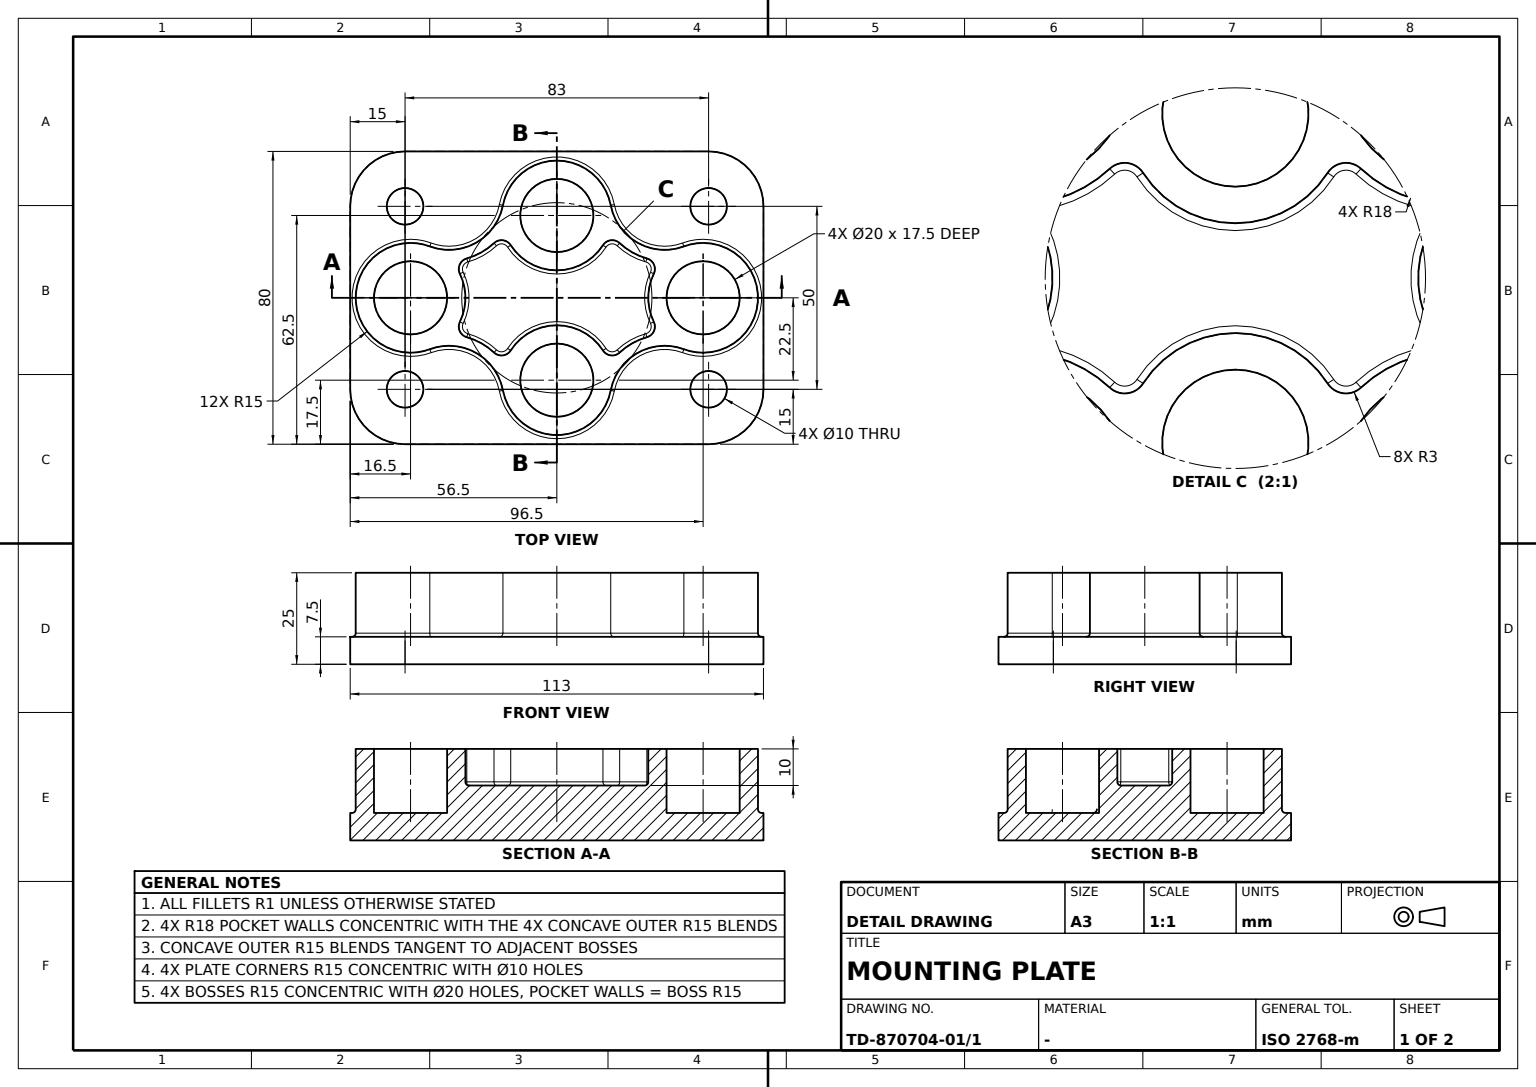
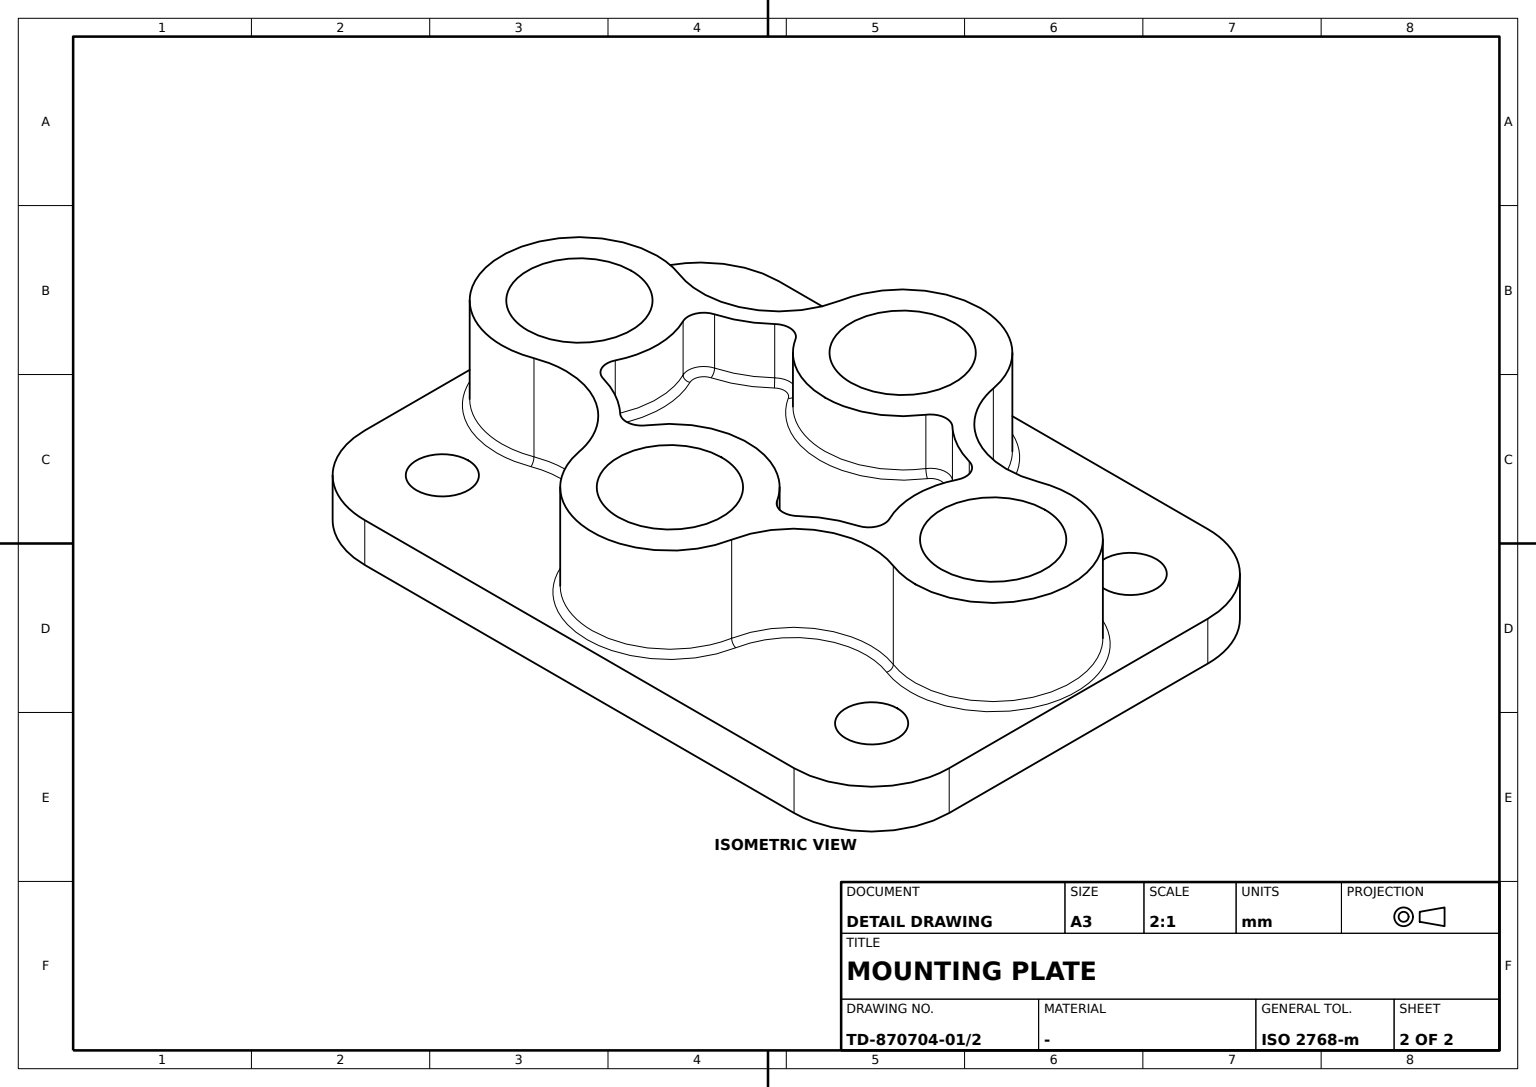
solid
v1 (-12.5,0,7.5)
v2 (-32.5,0,7.5)
e1 v1 v2 CIRCLE(AX(P(-22.5,0,7.5),D(0,0,-1),D(1,0,0)),10)
e2 v2 v1 CIRCLE(AX(P(-22.5,0,7.5),D(0,0,-1),D(1,0,0)),10)
face PLANE(AX(P(-22.5,0,7.5),D(0,0,1),D(1,0,0))) [-e1 -e2]
v3 (-14.213683,-16.498306,15)
v4 (-9.796458,-24.351149,15)
e3 v3 v4 CIRCLE(AX(P(-28.092789,-29.474069,15),D(0,0,-1),D(1,0,0)),19)
v5 (-14.944162,-17.181241,16)
e4 v5 v3 CIRCLE(AX(P(-14.213683,-16.498306,16),D(0.682934889,-0.730479252,0),D(0.730479252,0.682934889,0)),1)
v6 (-10.759423,-24.620776,16)
e5 v6 v5 CIRCLE(AX(P(-28.092789,-29.474069,16),D(0,0,1),D(1,0,0)),18)
e6 v6 v4 CIRCLE(AX(P(-9.796458,-24.351149,16),D(0.269627355,-0.962964739,0),D(0.962964739,0.269627355,0)),1)
face TORUS(AX(P(-28.092789,-29.474069,16),D(0,0,1),D(1,0,0)),19,1) rev [-e3 -e4 -e5 e6]
v7 (-6.996026,-25.610573,15)
v8 (6.996026,-25.610573,15)
e7 v7 v8 CIRCLE(AX(P(0,-40,15),D(0,0,-1),D(1,0,0)),16)
v9 (-6.558774,-26.509912,16)
e8 v9 v7 CIRCLE(AX(P(-6.996026,-25.610573,16),D(0.899339218,0.437251611,0),D(-0.437251611,0.899339218,0)),1)
v10 (6.558774,-26.509912,16)
e9 v10 v9 CIRCLE(AX(P(0,-40,16),D(0,0,1),D(1,0,0)),15)
e10 v10 v8 CIRCLE(AX(P(6.996026,-25.610573,16),D(0.899339218,-0.437251611,0),D(0.437251611,0.899339218,0)),1)
face TORUS(AX(P(0,-40,16),D(0,0,1),D(1,0,0)),16,1) rev [-e7 -e8 -e9 e10]
v11 (-25,56.5,0)
v12 (-25,56.5,7.5)
e11 v11 v12 LINE
v13 (25,56.5,7.5)
e12 v13 v12 LINE
v14 (25,56.5,0)
e13 v13 v14 LINE
e14 v14 v11 LINE
face PLANE(AX(P(40,56.5,7.5),D(0,-1,0),D(1,0,0))) rev [e11 -e12 e13 e14]
v15 (-10,40,25)
v16 (-10,40,7.5)
e15 v15 v16 LINE
v17 (10,40,25)
e16 v15 v17 CIRCLE(AX(P(0,40,25),D(0,0,1),D(1,0,0)),10)
v18 (10,40,7.5)
e17 v18 v17 LINE
e18 v18 v16 CIRCLE(AX(P(0,40,7.5),D(0,0,-1),D(1,0,0)),10)
face CYL(AX(P(0,40,7.5),D(0,0,1),D(1,0,0)),10) rev [-e15 e16 -e17 e18]
v19 (-40,-41.5,0)
v20 (-40,-41.5,7.5)
e19 v19 v20 LINE
v21 (-25,-56.5,0)
e20 v21 v19 CIRCLE(AX(P(-25,-41.5,0),D(0,0,-1),D(1,0,0)),15)
v22 (-25,-56.5,7.5)
e21 v22 v21 LINE
e22 v20 v22 CIRCLE(AX(P(-25,-41.5,7.5),D(0,0,1),D(1,0,0)),15)
face CYL(AX(P(-25,-41.5,7.5),D(0,0,-1),D(-1,0,0)),15) [-e19 -e20 -e21 -e22]
v23 (13.092789,-29.474069,8.5)
v24 (25.296394,-14.737034,8.5)
e23 v23 v24 CIRCLE(AX(P(28.092789,-29.474069,8.5),D(0,0,-1),D(1,0,0)),15)
v25 (25.296394,-14.737034,25)
e24 v25 v24 LINE
v26 (13.092789,-29.474069,25)
e25 v26 v25 CIRCLE(AX(P(28.092789,-29.474069,25),D(0,0,-1),D(-1,0,0)),15)
e26 v26 v23 LINE
face CYL(AX(P(28.092789,-29.474069,25),D(0,0,-1),D(-1,0,0)),15) rev [e23 -e24 -e25 e26]
v27 (-14.046394,34.737034,8.5)
v28 (-13.092789,29.474069,8.5)
e27 v27 v28 CIRCLE(AX(P(-28.092789,29.474069,8.5),D(0,0,-1),D(1,0,0)),15)
v29 (-25.296394,14.737034,8.5)
e28 v28 v29 CIRCLE(AX(P(-28.092789,29.474069,8.5),D(0,0,-1),D(1,0,0)),15)
v30 (-25.296394,14.737034,25)
e29 v30 v29 LINE
v31 (-14.046394,34.737034,25)
e30 v31 v30 CIRCLE(AX(P(-28.092789,29.474069,25),D(0,0,-1),D(-1,0,0)),15)
e31 v31 v27 LINE
face CYL(AX(P(-28.092789,29.474069,25),D(0,0,-1),D(-1,0,0)),15) rev [e27 e28 -e29 -e30 e31]
v32 (-20,-41.5,0)
v33 (-30,-41.5,0)
e32 v32 v33 CIRCLE(AX(P(-25,-41.5,0),D(0,0,1),D(-1,0,0)),5)
v34 (-20,-41.5,7.5)
e33 v32 v34 LINE
v35 (-30,-41.5,7.5)
e34 v34 v35 CIRCLE(AX(P(-25,-41.5,7.5),D(0,0,1),D(-1,0,0)),5)
e35 v35 v33 LINE
face CYL(AX(P(-25,-41.5,0),D(0,0,1),D(1,0,0)),5) rev [-e32 e33 e34 e35]
v36 (25.482821,-15.719503,7.5)
e36 v36 v24 CIRCLE(AX(P(25.482821,-15.719503,8.5),D(0.982468951,0.186426284,0),D(-0.186426284,0.982468951,0)),1)
v37 (38.5,0,7.5)
e37 v37 v36 CIRCLE(AX(P(22.5,0,7.5),D(0,0,-1),D(1,0,0)),16)
v38 (37.5,0,8.5)
e38 v38 v37 CIRCLE(AX(P(38.5,0,8.5),D(0,-1,0),D(0,0,-1)),1)
e39 v24 v38 CIRCLE(AX(P(22.5,0,8.5),D(0,0,1),D(1,0,0)),15)
face TORUS(AX(P(22.5,0,8.5),D(0,0,1),D(1,0,0)),16,1) rev [-e36 -e37 -e38 -e39]
v39 (-15,-40,8.5)
v40 (15,-40,8.5)
e40 v39 v40 CIRCLE(AX(P(0,-40,8.5),D(0,0,1),D(1,0,0)),15)
v41 (-16,-40,7.5)
e41 v39 v41 CIRCLE(AX(P(-16,-40,8.5),D(0,1,0),D(-1,0,0)),1)
v42 (16,-40,7.5)
e42 v42 v41 CIRCLE(AX(P(0,-40,7.5),D(0,0,-1),D(1,0,0)),16)
e43 v40 v42 CIRCLE(AX(P(16,-40,8.5),D(0,-1,0),D(0,0,-1)),1)
face TORUS(AX(P(0,-40,8.5),D(0,0,1),D(1,0,0)),16,1) rev [-e40 e41 -e42 -e43]
v43 (30,41.5,7.5)
v44 (20,41.5,7.5)
e44 v43 v44 CIRCLE(AX(P(25,41.5,7.5),D(0,0,1),D(-1,0,0)),5)
e45 v44 v43 CIRCLE(AX(P(25,41.5,7.5),D(0,0,1),D(-1,0,0)),5)
v45 (30,-41.5,7.5)
v46 (20,-41.5,7.5)
e46 v45 v46 CIRCLE(AX(P(25,-41.5,7.5),D(0,0,1),D(-1,0,0)),5)
e47 v46 v45 CIRCLE(AX(P(25,-41.5,7.5),D(0,0,1),D(-1,0,0)),5)
v47 (25,-56.5,7.5)
v48 (40,-41.5,7.5)
e48 v47 v48 CIRCLE(AX(P(25,-41.5,7.5),D(0,0,1),D(1,0,0)),15)
v49 (40,41.5,7.5)
e49 v48 v49 LINE
e50 v49 v13 CIRCLE(AX(P(25,41.5,7.5),D(0,0,1),D(1,0,0)),15)
v50 (-40,41.5,7.5)
e51 v12 v50 CIRCLE(AX(P(-25,41.5,7.5),D(0,0,1),D(1,0,0)),15)
e52 v50 v20 LINE
e53 v22 v47 LINE
v51 (-20,41.5,7.5)
v52 (-30,41.5,7.5)
e54 v51 v52 CIRCLE(AX(P(-25,41.5,7.5),D(0,0,1),D(-1,0,0)),5)
e55 v52 v51 CIRCLE(AX(P(-25,41.5,7.5),D(0,0,1),D(-1,0,0)),5)
e56 v35 v34 CIRCLE(AX(P(-25,-41.5,7.5),D(0,0,1),D(-1,0,0)),5)
v53 (16,40,7.5)
v54 (14.982821,34.38617,7.5)
e57 v53 v54 CIRCLE(AX(P(0,40,7.5),D(0,0,-1),D(1,0,0)),16)
v55 (25.482821,15.719503,7.5)
e58 v54 v55 CIRCLE(AX(P(28.092789,29.474069,7.5),D(0,0,1),D(1,0,0)),14)
e59 v55 v37 CIRCLE(AX(P(22.5,0,7.5),D(0,0,-1),D(1,0,0)),16)
v56 (14.982821,-34.38617,7.5)
e60 v36 v56 CIRCLE(AX(P(28.092789,-29.474069,7.5),D(0,0,1),D(1,0,0)),14)
e61 v56 v42 CIRCLE(AX(P(0,-40,7.5),D(0,0,-1),D(1,0,0)),16)
v57 (-14.982821,-34.38617,7.5)
e62 v41 v57 CIRCLE(AX(P(0,-40,7.5),D(0,0,-1),D(1,0,0)),16)
v58 (-14.092789,-29.474069,7.5)
e63 v57 v58 CIRCLE(AX(P(-28.092789,-29.474069,7.5),D(0,0,1),D(1,0,0)),14)
v59 (-25.482821,-15.719503,7.5)
e64 v58 v59 CIRCLE(AX(P(-28.092789,-29.474069,7.5),D(0,0,1),D(1,0,0)),14)
v60 (-25.482821,15.719503,7.5)
e65 v59 v60 CIRCLE(AX(P(-22.5,0,7.5),D(0,0,-1),D(1,0,0)),16)
v61 (-14.092789,29.474069,7.5)
e66 v60 v61 CIRCLE(AX(P(-28.092789,29.474069,7.5),D(0,0,1),D(1,0,0)),14)
v62 (-14.982821,34.38617,7.5)
e67 v61 v62 CIRCLE(AX(P(-28.092789,29.474069,7.5),D(0,0,1),D(1,0,0)),14)
v63 (-16,40,7.5)
e68 v62 v63 CIRCLE(AX(P(0,40,7.5),D(0,0,-1),D(1,0,0)),16)
e69 v63 v53 CIRCLE(AX(P(0,40,7.5),D(0,0,-1),D(1,0,0)),16)
face PLANE(AX(P(0,0,7.5),D(0,0,1),D(1,0,0))) [-e44 -e45] [-e46 -e47] [e48 e49 e50 e12 e51 e52 e22 e53] [-e54 -e55] [-e34 -e56] [e57 e58 e59 e37 e60 e61 e42 e62 e63 e64 e65 e66 e67 e68 e69]
v64 (-20,41.5,0)
e70 v64 v51 LINE
v65 (-30,41.5,0)
e71 v65 v64 CIRCLE(AX(P(-25,41.5,0),D(0,0,1),D(-1,0,0)),5)
e72 v52 v65 LINE
face CYL(AX(P(-25,41.5,0),D(0,0,1),D(1,0,0)),5) rev [-e70 -e71 -e72 e55]
v66 (14.37727,-12.610363,16)
v67 (15.752724,-15.132436,16)
e73 v66 v67 CIRCLE(AX(P(12.752724,-15.132436,16),D(0,0,-1),D(1,0,0)),3)
v68 (15.752724,-15.132436,25)
e74 v67 v68 LINE
v69 (14.37727,-12.610363,25)
e75 v68 v69 CIRCLE(AX(P(12.752724,-15.132436,25),D(0,0,1),D(1,0,0)),3)
e76 v69 v66 LINE
face CYL(AX(P(12.752724,-15.132436,15),D(0,0,1),D(1,0,0)),3) rev [e73 e74 e75 e76]
v70 (10.759423,-24.620776,25)
v71 (14.944162,-17.181241,25)
e77 v70 v71 CIRCLE(AX(P(28.092789,-29.474069,25),D(0,0,-1),D(1,0,0)),18)
v72 (14.944162,-17.181241,16)
e78 v71 v72 LINE
v73 (10.759423,-24.620776,16)
e79 v72 v73 CIRCLE(AX(P(28.092789,-29.474069,16),D(0,0,1),D(1,0,0)),18)
e80 v70 v73 LINE
face CYL(AX(P(28.092789,-29.474069,15),D(0,0,1),D(1,0,0)),18) [e77 e78 e79 -e80]
v74 (15,40,8.5)
v75 (-15,40,8.5)
e81 v74 v75 CIRCLE(AX(P(0,40,8.5),D(0,0,1),D(1,0,0)),15)
e82 v74 v53 CIRCLE(AX(P(16,40,8.5),D(0,-1,0),D(0,0,-1)),1)
e83 v75 v63 CIRCLE(AX(P(-16,40,8.5),D(0,1,0),D(-1,0,0)),1)
face TORUS(AX(P(0,40,8.5),D(0,0,1),D(1,0,0)),16,1) rev [-e81 e82 -e69 -e83]
v76 (-37.5,0,8.5)
e84 v29 v76 CIRCLE(AX(P(-22.5,0,8.5),D(0,0,1),D(1,0,0)),15)
v77 (-37.5,0,25)
e85 v77 v76 LINE
e86 v30 v77 CIRCLE(AX(P(-22.5,0,25),D(0,0,1),D(-1,0,0)),15)
face CYL(AX(P(-22.5,0,25),D(0,0,-1),D(-1,0,0)),15) [e84 -e85 -e86 e29]
v78 (-15,-40,25)
e87 v78 v39 LINE
v79 (15,-40,25)
e88 v79 v40 LINE
e89 v78 v79 CIRCLE(AX(P(0,-40,25),D(0,0,1),D(-1,0,0)),15)
face CYL(AX(P(0,-40,25),D(0,0,-1),D(-1,0,0)),15) [e87 e40 -e88 -e89]
v80 (-10,-40,25)
v81 (-10,-40,7.5)
e90 v80 v81 LINE
v82 (10,-40,7.5)
e91 v81 v82 CIRCLE(AX(P(0,-40,7.5),D(0,0,-1),D(1,0,0)),10)
v83 (10,-40,25)
e92 v82 v83 LINE
e93 v83 v80 CIRCLE(AX(P(0,-40,25),D(0,0,1),D(1,0,0)),10)
face CYL(AX(P(0,-40,7.5),D(0,0,1),D(1,0,0)),10) rev [e90 e91 e92 e93]
e94 v33 v32 CIRCLE(AX(P(-25,-41.5,0),D(0,0,1),D(-1,0,0)),5)
face CYL(AX(P(-25,-41.5,0),D(0,0,1),D(1,0,0)),5) rev [-e94 -e35 e56 -e33]
v84 (10.759423,24.620776,16)
v85 (14.944162,17.181241,16)
e95 v84 v85 CIRCLE(AX(P(28.092789,29.474069,16),D(0,0,1),D(1,0,0)),18)
v86 (9.796458,24.351149,15)
e96 v86 v84 CIRCLE(AX(P(9.796458,24.351149,16),D(0.269627355,-0.962964739,0),D(0.962964739,0.269627355,0)),1)
v87 (14.213683,16.498306,15)
e97 v87 v86 CIRCLE(AX(P(28.092789,29.474069,15),D(0,0,-1),D(1,0,0)),19)
e98 v87 v85 CIRCLE(AX(P(14.213683,16.498306,16),D(0.682934889,-0.730479252,0),D(0.730479252,0.682934889,0)),1)
face TORUS(AX(P(28.092789,29.474069,16),D(0,0,1),D(1,0,0)),19,1) rev [-e95 -e96 -e97 e98]
e99 v62 v27 CIRCLE(AX(P(-14.982821,34.38617,8.5),D(0.350864382,-0.936426284,0),D(0.936426284,0.350864382,0)),1)
e100 v75 v27 CIRCLE(AX(P(0,40,8.5),D(0,0,1),D(1,0,0)),15)
face TORUS(AX(P(0,40,8.5),D(0,0,1),D(1,0,0)),16,1) rev [e83 -e68 e99 -e100]
e101 v61 v28 CIRCLE(AX(P(-14.092789,29.474069,8.5),D(0,-1,0),D(0,0,-1)),1)
e102 v29 v60 CIRCLE(AX(P(-25.482821,15.719503,8.5),D(0.982468951,0.186426284,0),D(-0.186426284,0.982468951,0)),1)
face TORUS(AX(P(-28.092789,29.474069,8.5),D(0,0,1),D(1,0,0)),14,1) rev [-e101 -e66 -e102 -e28]
v88 (40,-41.5,0)
e103 v48 v88 LINE
v89 (40,41.5,0)
e104 v88 v89 LINE
e105 v89 v49 LINE
face PLANE(AX(P(40,-56.5,7.5),D(-1,0,0),D(0,-1,0))) rev [e103 e104 e105 -e49]
e106 v80 v83 CIRCLE(AX(P(0,-40,25),D(0,0,1),D(1,0,0)),10)
e107 v82 v81 CIRCLE(AX(P(0,-40,7.5),D(0,0,-1),D(1,0,0)),10)
face CYL(AX(P(0,-40,7.5),D(0,0,1),D(1,0,0)),10) rev [-e90 e106 -e92 e107]
v90 (-6.558774,26.509912,16)
v91 (6.558774,26.509912,16)
e108 v90 v91 CIRCLE(AX(P(0,40,16),D(0,0,1),D(1,0,0)),15)
v92 (-6.996026,25.610573,15)
e109 v92 v90 CIRCLE(AX(P(-6.996026,25.610573,16),D(0.899339218,-0.437251611,0),D(0.437251611,0.899339218,0)),1)
v93 (6.996026,25.610573,15)
e110 v93 v92 CIRCLE(AX(P(0,40,15),D(0,0,-1),D(1,0,0)),16)
e111 v93 v91 CIRCLE(AX(P(6.996026,25.610573,16),D(0.899339218,0.437251611,0),D(-0.437251611,0.899339218,0)),1)
face TORUS(AX(P(0,40,16),D(0,0,1),D(1,0,0)),16,1) rev [-e108 -e109 -e110 e111]
v94 (20,41.5,0)
e112 v44 v94 LINE
v95 (30,41.5,0)
e113 v95 v43 LINE
e114 v94 v95 CIRCLE(AX(P(25,41.5,0),D(0,0,1),D(-1,0,0)),5)
face CYL(AX(P(25,41.5,0),D(0,0,1),D(1,0,0)),5) rev [-e112 e45 -e113 -e114]
v96 (-40,41.5,0)
e115 v50 v96 LINE
e116 v96 v19 LINE
face PLANE(AX(P(-40,56.5,7.5),D(1,0,0),D(0,1,0))) rev [-e52 e115 e116 e19]
v97 (14.046394,-34.737034,8.5)
e117 v97 v23 CIRCLE(AX(P(28.092789,-29.474069,8.5),D(0,0,-1),D(1,0,0)),15)
e118 v97 v56 CIRCLE(AX(P(14.982821,-34.38617,8.5),D(0.350864382,-0.936426284,0),D(0.936426284,0.350864382,0)),1)
face TORUS(AX(P(28.092789,-29.474069,8.5),D(0,0,1),D(1,0,0)),14,1) rev [-e60 e36 -e23 -e117 e118]
v98 (6.558774,26.509912,25)
e119 v98 v91 LINE
v99 (-6.558774,26.509912,25)
e120 v98 v99 CIRCLE(AX(P(0,40,25),D(0,0,-1),D(1,0,0)),15)
e121 v99 v90 LINE
face CYL(AX(P(0,40,15),D(0,0,1),D(1,0,0)),15) [-e119 e120 e121 e108]
v100 (-7.5,0,16)
v101 (-7.5,0,25)
e122 v100 v101 LINE
v102 (-14.37727,12.610363,16)
e123 v100 v102 CIRCLE(AX(P(-22.5,0,16),D(0,0,1),D(1,0,0)),15)
v103 (-14.37727,12.610363,25)
e124 v103 v102 LINE
e125 v103 v101 CIRCLE(AX(P(-22.5,0,25),D(0,0,-1),D(1,0,0)),15)
face CYL(AX(P(-22.5,0,15),D(0,0,1),D(1,0,0)),15) [-e122 e123 -e124 e125]
v104 (12.5,0,25)
v105 (32.5,0,25)
e126 v104 v105 CIRCLE(AX(P(22.5,0,25),D(0,0,1),D(1,0,0)),10)
e127 v105 v104 CIRCLE(AX(P(22.5,0,25),D(0,0,1),D(1,0,0)),10)
v106 (-14.046394,-34.737034,25)
e128 v106 v78 CIRCLE(AX(P(0,-40,25),D(0,0,1),D(-1,0,0)),15)
v107 (14.046394,-34.737034,25)
e129 v79 v107 CIRCLE(AX(P(0,-40,25),D(0,0,1),D(-1,0,0)),15)
e130 v107 v26 CIRCLE(AX(P(28.092789,-29.474069,25),D(0,0,-1),D(-1,0,0)),15)
v108 (25.296394,14.737034,25)
e131 v25 v108 CIRCLE(AX(P(22.5,0,25),D(0,0,1),D(-1,0,0)),15)
v109 (13.092789,29.474069,25)
e132 v108 v109 CIRCLE(AX(P(28.092789,29.474069,25),D(0,0,-1),D(-1,0,0)),15)
v110 (14.046394,34.737034,25)
e133 v109 v110 CIRCLE(AX(P(28.092789,29.474069,25),D(0,0,-1),D(-1,0,0)),15)
v111 (15,40,25)
e134 v110 v111 CIRCLE(AX(P(0,40,25),D(0,0,1),D(-1,0,0)),15)
v112 (-15,40,25)
e135 v111 v112 CIRCLE(AX(P(0,40,25),D(0,0,1),D(-1,0,0)),15)
e136 v112 v31 CIRCLE(AX(P(0,40,25),D(0,0,1),D(-1,0,0)),15)
v113 (-25.296394,-14.737034,25)
e137 v77 v113 CIRCLE(AX(P(-22.5,0,25),D(0,0,1),D(-1,0,0)),15)
e138 v113 v106 CIRCLE(AX(P(-28.092789,-29.474069,25),D(0,0,-1),D(-1,0,0)),15)
v114 (15.752724,15.132436,25)
v115 (14.944162,17.181241,25)
e139 v114 v115 CIRCLE(AX(P(12.752724,15.132436,25),D(0,0,1),D(1,0,0)),3)
v116 (14.37727,12.610363,25)
e140 v116 v114 CIRCLE(AX(P(12.752724,15.132436,25),D(0,0,1),D(1,0,0)),3)
e141 v69 v116 CIRCLE(AX(P(22.5,0,25),D(0,0,-1),D(1,0,0)),15)
e142 v71 v68 CIRCLE(AX(P(12.752724,-15.132436,25),D(0,0,1),D(1,0,0)),3)
v117 (6.558774,-26.509912,25)
e143 v117 v70 CIRCLE(AX(P(7.870529,-23.811894,25),D(0,0,1),D(1,0,0)),3)
v118 (-6.558774,-26.509912,25)
e144 v118 v117 CIRCLE(AX(P(0,-40,25),D(0,0,-1),D(1,0,0)),15)
v119 (-10.759423,-24.620776,25)
e145 v119 v118 CIRCLE(AX(P(-7.870529,-23.811894,25),D(0,0,1),D(1,0,0)),3)
v120 (-14.944162,-17.181241,25)
e146 v120 v119 CIRCLE(AX(P(-28.092789,-29.474069,25),D(0,0,-1),D(1,0,0)),18)
v121 (-14.37727,-12.610363,25)
e147 v121 v120 CIRCLE(AX(P(-12.752724,-15.132436,25),D(0,0,1),D(1,0,0)),3)
e148 v101 v121 CIRCLE(AX(P(-22.5,0,25),D(0,0,-1),D(1,0,0)),15)
v122 (-14.944162,17.181241,25)
e149 v122 v103 CIRCLE(AX(P(-12.752724,15.132436,25),D(0,0,1),D(1,0,0)),3)
v123 (-10.759423,24.620776,25)
e150 v123 v122 CIRCLE(AX(P(-28.092789,29.474069,25),D(0,0,-1),D(1,0,0)),18)
e151 v99 v123 CIRCLE(AX(P(-7.870529,23.811894,25),D(0,0,1),D(1,0,0)),3)
v124 (10.759423,24.620776,25)
e152 v124 v98 CIRCLE(AX(P(7.870529,23.811894,25),D(0,0,1),D(1,0,0)),3)
e153 v115 v124 CIRCLE(AX(P(28.092789,29.474069,25),D(0,0,-1),D(1,0,0)),18)
v125 (-32.5,0,25)
v126 (-12.5,0,25)
e154 v125 v126 CIRCLE(AX(P(-22.5,0,25),D(0,0,1),D(1,0,0)),10)
e155 v126 v125 CIRCLE(AX(P(-22.5,0,25),D(0,0,1),D(1,0,0)),10)
e156 v17 v15 CIRCLE(AX(P(0,40,25),D(0,0,1),D(1,0,0)),10)
face PLANE(AX(P(-25.296394,-14.737034,25),D(0,0,1),D(1,0,0))) [-e126 -e127] [e128 e89 e129 e130 e25 e131 e132 e133 e134 e135 e136 e30 e86 e137 e138] [-e139 -e140 -e141 -e75 -e142 -e77 -e143 -e144 -e145 -e146 -e147 -e148 -e125 -e149 -e150 -e151 -e120 -e152 -e153] [-e154 -e155] [-e93 -e106] [-e156 -e16]
e157 v16 v18 CIRCLE(AX(P(0,40,7.5),D(0,0,-1),D(1,0,0)),10)
face PLANE(AX(P(0,40,7.5),D(0,0,1),D(1,0,0))) [-e18 -e157]
v127 (-14.213683,16.498306,15)
v128 (-14.944162,17.181241,16)
e158 v127 v128 CIRCLE(AX(P(-14.213683,16.498306,16),D(0.682934889,0.730479252,0),D(-0.730479252,0.682934889,0)),1)
e159 v102 v128 CIRCLE(AX(P(-12.752724,15.132436,16),D(0,0,-1),D(1,0,0)),3)
v129 (-13.835755,13.451054,15)
e160 v102 v129 CIRCLE(AX(P(-13.835755,13.451054,16),D(0.840690882,-0.54151532,0),D(0.54151532,0.840690882,0)),1)
e161 v127 v129 CIRCLE(AX(P(-12.752724,15.132436,15),D(0,0,1),D(1,0,0)),2)
face TORUS(AX(P(-12.752724,15.132436,16),D(0,0,1),D(1,0,0)),2,1) rev [e158 -e159 e160 -e161]
e162 v64 v65 CIRCLE(AX(P(-25,41.5,0),D(0,0,1),D(-1,0,0)),5)
face CYL(AX(P(-25,41.5,0),D(0,0,1),D(1,0,0)),5) rev [-e162 e70 e54 e72]
v130 (13.835755,13.451054,15)
v131 (14.37727,12.610363,16)
e163 v130 v131 CIRCLE(AX(P(13.835755,13.451054,16),D(-0.840690882,-0.54151532,0),D(0.54151532,-0.840690882,0)),1)
v132 (15.752724,15.132436,16)
e164 v132 v131 CIRCLE(AX(P(12.752724,15.132436,16),D(0,0,-1),D(1,0,0)),3)
v133 (14.752724,15.132436,15)
e165 v133 v132 CIRCLE(AX(P(14.752724,15.132436,16),D(0,-1,0),D(0,0,-1)),1)
e166 v130 v133 CIRCLE(AX(P(12.752724,15.132436,15),D(0,0,1),D(1,0,0)),2)
face TORUS(AX(P(12.752724,15.132436,16),D(0,0,1),D(1,0,0)),2,1) rev [e163 -e164 -e165 -e166]
v134 (-10.759423,24.620776,16)
e167 v123 v134 LINE
e168 v134 v90 CIRCLE(AX(P(-7.870529,23.811894,16),D(0,0,-1),D(1,0,0)),3)
face CYL(AX(P(-7.870529,23.811894,15),D(0,0,1),D(1,0,0)),3) rev [e151 e167 e168 -e121]
e169 v117 v10 LINE
e170 v73 v10 CIRCLE(AX(P(7.870529,-23.811894,16),D(0,0,-1),D(1,0,0)),3)
face CYL(AX(P(7.870529,-23.811894,15),D(0,0,1),D(1,0,0)),3) rev [-e169 e143 e80 e170]
v135 (-14.046394,-34.737034,8.5)
e171 v106 v135 LINE
e172 v135 v39 CIRCLE(AX(P(0,-40,8.5),D(0,0,1),D(1,0,0)),15)
face CYL(AX(P(0,-40,25),D(0,0,-1),D(-1,0,0)),15) [-e87 -e128 e171 e172]
e173 v125 v2 LINE
e174 v1 v126 LINE
face CYL(AX(P(-22.5,0,7.5),D(0,0,1),D(1,0,0)),10) rev [e173 e2 e174 e155]
e175 v112 v75 LINE
e176 v111 v74 LINE
face CYL(AX(P(0,40,25),D(0,0,-1),D(-1,0,0)),15) [e81 -e175 -e135 e176]
v136 (-9.796458,24.351149,15)
e177 v136 v134 CIRCLE(AX(P(-9.796458,24.351149,16),D(0.269627355,0.962964739,0),D(-0.962964739,0.269627355,0)),1)
e178 v92 v136 CIRCLE(AX(P(-7.870529,23.811894,15),D(0,0,1),D(1,0,0)),2)
face TORUS(AX(P(-7.870529,23.811894,16),D(0,0,1),D(1,0,0)),2,1) rev [e109 -e168 -e177 -e178]
e179 v132 v114 LINE
e180 v116 v131 LINE
face CYL(AX(P(12.752724,15.132436,15),D(0,0,1),D(1,0,0)),3) rev [e140 -e179 e164 -e180]
v137 (-14.37727,-12.610363,16)
v138 (-13.835755,-13.451054,15)
e181 v137 v138 CIRCLE(AX(P(-13.835755,-13.451054,16),D(-0.840690882,-0.54151532,0),D(0.54151532,-0.840690882,0)),1)
e182 v5 v137 CIRCLE(AX(P(-12.752724,-15.132436,16),D(0,0,-1),D(1,0,0)),3)
e183 v138 v3 CIRCLE(AX(P(-12.752724,-15.132436,15),D(0,0,1),D(1,0,0)),2)
face TORUS(AX(P(-12.752724,-15.132436,16),D(0,0,1),D(1,0,0)),2,1) rev [-e181 -e182 e4 -e183]
e184 v86 v93 CIRCLE(AX(P(7.870529,23.811894,15),D(0,0,1),D(1,0,0)),2)
e185 v91 v84 CIRCLE(AX(P(7.870529,23.811894,16),D(0,0,-1),D(1,0,0)),3)
face TORUS(AX(P(7.870529,23.811894,16),D(0,0,1),D(1,0,0)),2,1) rev [-e111 -e184 e96 -e185]
v139 (-6.5,0,15)
e186 v100 v139 CIRCLE(AX(P(-6.5,0,16),D(0,-1,0),D(0,0,-1)),1)
e187 v129 v139 CIRCLE(AX(P(-22.5,0,15),D(0,0,-1),D(1,0,0)),16)
face TORUS(AX(P(-22.5,0,16),D(0,0,1),D(1,0,0)),16,1) rev [-e123 e186 -e187 -e160]
v140 (14.046394,34.737034,8.5)
e188 v54 v140 CIRCLE(AX(P(14.982821,34.38617,8.5),D(0.350864382,0.936426284,0),D(-0.936426284,0.350864382,0)),1)
v141 (13.092789,29.474069,8.5)
e189 v141 v140 CIRCLE(AX(P(28.092789,29.474069,8.5),D(0,0,-1),D(1,0,0)),15)
v142 (25.296394,14.737034,8.5)
e190 v142 v141 CIRCLE(AX(P(28.092789,29.474069,8.5),D(0,0,-1),D(1,0,0)),15)
e191 v55 v142 CIRCLE(AX(P(25.482821,15.719503,8.5),D(-0.982468951,0.186426284,0),D(-0.186426284,-0.982468951,0)),1)
face TORUS(AX(P(28.092789,29.474069,8.5),D(0,0,1),D(1,0,0)),14,1) rev [e188 -e189 -e190 -e191 -e58]
face CYL(AX(P(-22.5,0,7.5),D(0,0,1),D(1,0,0)),10) rev [e154 -e174 e1 -e173]
e192 v115 v85 LINE
e193 v85 v132 CIRCLE(AX(P(12.752724,15.132436,16),D(0,0,-1),D(1,0,0)),3)
face CYL(AX(P(12.752724,15.132436,15),D(0,0,1),D(1,0,0)),3) rev [e179 e139 e192 e193]
v143 (20,-41.5,0)
e194 v46 v143 LINE
v144 (30,-41.5,0)
e195 v144 v143 CIRCLE(AX(P(25,-41.5,0),D(0,0,1),D(-1,0,0)),5)
e196 v144 v45 LINE
face CYL(AX(P(25,-41.5,0),D(0,0,1),D(1,0,0)),5) rev [e46 e194 -e195 e196]
e197 v40 v97 CIRCLE(AX(P(0,-40,8.5),D(0,0,1),D(1,0,0)),15)
face TORUS(AX(P(0,-40,8.5),D(0,0,1),D(1,0,0)),16,1) rev [-e118 -e197 e43 -e61]
v145 (-25.296394,-14.737034,8.5)
v146 (-13.092789,-29.474069,8.5)
e198 v145 v146 CIRCLE(AX(P(-28.092789,-29.474069,8.5),D(0,0,-1),D(1,0,0)),15)
e199 v145 v59 CIRCLE(AX(P(-25.482821,-15.719503,8.5),D(-0.982468951,0.186426284,0),D(-0.186426284,-0.982468951,0)),1)
e200 v58 v146 CIRCLE(AX(P(-14.092789,-29.474069,8.5),D(0,-1,0),D(0,0,-1)),1)
face TORUS(AX(P(-28.092789,-29.474069,8.5),D(0,0,1),D(1,0,0)),14,1) rev [-e198 e199 -e64 e200]
e201 v107 v97 LINE
face CYL(AX(P(0,-40,25),D(0,0,-1),D(-1,0,0)),15) [-e129 e88 e197 -e201]
e202 v76 v145 CIRCLE(AX(P(-22.5,0,8.5),D(0,0,1),D(1,0,0)),15)
face TORUS(AX(P(-22.5,0,8.5),D(0,0,1),D(1,0,0)),16,1) rev [-e84 e102 -e65 -e199 -e202]
e203 v121 v137 LINE
e204 v137 v100 CIRCLE(AX(P(-22.5,0,16),D(0,0,1),D(1,0,0)),15)
face CYL(AX(P(-22.5,0,15),D(0,0,1),D(1,0,0)),15) [e148 e203 e204 e122]
e205 v38 v142 CIRCLE(AX(P(22.5,0,8.5),D(0,0,1),D(1,0,0)),15)
face TORUS(AX(P(22.5,0,8.5),D(0,0,1),D(1,0,0)),16,1) rev [e191 -e205 e38 -e59]
face CYL(AX(P(28.092789,-29.474069,25),D(0,0,-1),D(-1,0,0)),15) rev [-e26 -e130 e201 e117]
v147 (14.213683,-16.498306,15)
e206 v72 v147 CIRCLE(AX(P(14.213683,-16.498306,16),D(0.682934889,0.730479252,0),D(-0.730479252,0.682934889,0)),1)
v148 (9.796458,-24.351149,15)
e207 v148 v147 CIRCLE(AX(P(28.092789,-29.474069,15),D(0,0,-1),D(1,0,0)),19)
e208 v73 v148 CIRCLE(AX(P(9.796458,-24.351149,16),D(0.269627355,0.962964739,0),D(-0.962964739,0.269627355,0)),1)
face TORUS(AX(P(28.092789,-29.474069,16),D(0,0,1),D(1,0,0)),19,1) rev [e206 -e207 -e208 -e79]
e209 v113 v145 LINE
face CYL(AX(P(-22.5,0,25),D(0,0,-1),D(-1,0,0)),15) [-e137 e85 e202 -e209]
e210 v95 v94 CIRCLE(AX(P(25,41.5,0),D(0,0,1),D(-1,0,0)),5)
face CYL(AX(P(25,41.5,0),D(0,0,1),D(1,0,0)),5) rev [-e210 e113 e44 e112]
e211 v139 v138 CIRCLE(AX(P(-22.5,0,15),D(0,0,-1),D(1,0,0)),16)
face TORUS(AX(P(-22.5,0,16),D(0,0,1),D(1,0,0)),16,1) rev [-e186 -e204 e181 -e211]
v149 (12.5,0,7.5)
v150 (32.5,0,7.5)
e212 v149 v150 CIRCLE(AX(P(22.5,0,7.5),D(0,0,-1),D(1,0,0)),10)
e213 v150 v105 LINE
e214 v104 v149 LINE
face CYL(AX(P(22.5,0,7.5),D(0,0,1),D(1,0,0)),10) rev [e212 e213 e127 e214]
e215 v122 v128 LINE
e216 v128 v134 CIRCLE(AX(P(-28.092789,29.474069,16),D(0,0,1),D(1,0,0)),18)
face CYL(AX(P(-28.092789,29.474069,15),D(0,0,1),D(1,0,0)),18) [-e167 e150 e215 e216]
e217 v108 v142 LINE
face CYL(AX(P(22.5,0,25),D(0,0,-1),D(-1,0,0)),15) [-e131 e24 e39 e205 -e217]
e218 v67 v72 CIRCLE(AX(P(12.752724,-15.132436,16),D(0,0,-1),D(1,0,0)),3)
face CYL(AX(P(12.752724,-15.132436,15),D(0,0,1),D(1,0,0)),3) rev [-e74 e218 -e78 e142]
e219 v150 v149 CIRCLE(AX(P(22.5,0,7.5),D(0,0,-1),D(1,0,0)),10)
face PLANE(AX(P(22.5,0,7.5),D(0,0,1),D(1,0,0))) [-e219 -e212]
e220 v124 v84 LINE
face CYL(AX(P(7.870529,23.811894,15),D(0,0,1),D(1,0,0)),3) rev [e119 e185 -e220 e152]
e221 v96 v11 CIRCLE(AX(P(-25,41.5,0),D(0,0,-1),D(1,0,0)),15)
face CYL(AX(P(-25,41.5,7.5),D(0,0,-1),D(-1,0,0)),15) [-e221 -e115 -e51 -e11]
e222 v140 v74 CIRCLE(AX(P(0,40,8.5),D(0,0,1),D(1,0,0)),15)
face TORUS(AX(P(0,40,8.5),D(0,0,1),D(1,0,0)),16,1) rev [-e57 -e82 -e222 -e188]
e223 v118 v9 LINE
e224 v9 v6 CIRCLE(AX(P(-7.870529,-23.811894,16),D(0,0,-1),D(1,0,0)),3)
e225 v119 v6 LINE
face CYL(AX(P(-7.870529,-23.811894,15),D(0,0,1),D(1,0,0)),3) rev [e145 e223 e224 -e225]
e226 v131 v66 CIRCLE(AX(P(22.5,0,16),D(0,0,1),D(1,0,0)),15)
face CYL(AX(P(22.5,0,15),D(0,0,1),D(1,0,0)),15) [e180 e226 -e76 e141]
v151 (13.835755,-13.451054,15)
e227 v151 v66 CIRCLE(AX(P(13.835755,-13.451054,16),D(0.840690882,-0.54151532,0),D(0.54151532,0.840690882,0)),1)
e228 v151 v130 CIRCLE(AX(P(22.5,0,15),D(0,0,-1),D(1,0,0)),16)
face TORUS(AX(P(22.5,0,16),D(0,0,1),D(1,0,0)),16,1) rev [e227 -e226 -e163 -e228]
e229 v4 v7 CIRCLE(AX(P(-7.870529,-23.811894,15),D(0,0,1),D(1,0,0)),2)
face TORUS(AX(P(-7.870529,-23.811894,16),D(0,0,1),D(1,0,0)),2,1) rev [-e224 e8 -e229 -e6]
e230 v120 v5 LINE
face CYL(AX(P(-28.092789,-29.474069,15),D(0,0,1),D(1,0,0)),18) [e225 e5 -e230 e146]
e231 v109 v141 LINE
face CYL(AX(P(28.092789,29.474069,25),D(0,0,-1),D(-1,0,0)),15) rev [e217 e190 -e231 -e132]
v152 (25,-56.5,0)
e232 v152 v47 LINE
e233 v88 v152 CIRCLE(AX(P(25,-41.5,0),D(0,0,-1),D(1,0,0)),15)
face CYL(AX(P(25,-41.5,7.5),D(0,0,-1),D(-1,0,0)),15) [-e103 -e48 -e232 -e233]
face TORUS(AX(P(-28.092789,29.474069,8.5),D(0,0,1),D(1,0,0)),14,1) rev [e101 -e27 -e99 -e67]
e234 v133 v87 CIRCLE(AX(P(12.752724,15.132436,15),D(0,0,1),D(1,0,0)),2)
face TORUS(AX(P(12.752724,15.132436,16),D(0,0,1),D(1,0,0)),2,1) rev [-e98 -e234 e165 -e193]
face CYL(AX(P(-12.752724,-15.132436,15),D(0,0,1),D(1,0,0)),3) rev [e230 e182 -e203 e147]
v153 (14.752724,-15.132436,15)
e235 v153 v67 CIRCLE(AX(P(14.752724,-15.132436,16),D(0,-1,0),D(0,0,-1)),1)
e236 v147 v153 CIRCLE(AX(P(12.752724,-15.132436,15),D(0,0,1),D(1,0,0)),2)
face TORUS(AX(P(12.752724,-15.132436,16),D(0,0,1),D(1,0,0)),2,1) rev [-e206 -e218 -e235 -e236]
face CYL(AX(P(22.5,0,7.5),D(0,0,1),D(1,0,0)),10) rev [e126 -e213 e219 -e214]
e237 v136 v127 CIRCLE(AX(P(-28.092789,29.474069,15),D(0,0,-1),D(1,0,0)),19)
face TORUS(AX(P(-28.092789,29.474069,16),D(0,0,1),D(1,0,0)),19,1) rev [-e158 -e237 e177 -e216]
e238 v135 v57 CIRCLE(AX(P(-14.982821,-34.38617,8.5),D(0.350864382,0.936426284,0),D(-0.936426284,0.350864382,0)),1)
face TORUS(AX(P(0,-40,8.5),D(0,0,1),D(1,0,0)),16,1) rev [-e62 -e41 -e172 e238]
face CYL(AX(P(0,40,25),D(0,0,-1),D(-1,0,0)),15) [e175 e100 -e31 -e136]
face CYL(AX(P(0,-40,15),D(0,0,1),D(1,0,0)),15) [e169 e9 -e223 e144]
e239 v21 v152 LINE
face PLANE(AX(P(-40,-56.5,7.5),D(0,1,0),D(-1,0,0))) rev [e239 e232 -e53 e21]
e240 v153 v151 CIRCLE(AX(P(12.752724,-15.132436,15),D(0,0,1),D(1,0,0)),2)
face TORUS(AX(P(12.752724,-15.132436,16),D(0,0,1),D(1,0,0)),2,1) rev [-e73 -e227 -e240 e235]
e241 v8 v148 CIRCLE(AX(P(7.870529,-23.811894,15),D(0,0,1),D(1,0,0)),2)
face TORUS(AX(P(7.870529,-23.811894,16),D(0,0,1),D(1,0,0)),2,1) rev [-e241 -e10 -e170 e208]
face PLANE(AX(P(-20.422756,-22.303252,15),D(0,0,1),D(1,0,0))) [e211 e183 e3 e229 e7 e241 e207 e236 e240 e228 e166 e234 e97 e184 e110 e178 e237 e161 e187]
face CYL(AX(P(-12.752724,15.132436,15),D(0,0,1),D(1,0,0)),3) rev [e149 e124 e159 -e215]
e242 v143 v144 CIRCLE(AX(P(25,-41.5,0),D(0,0,1),D(-1,0,0)),5)
face CYL(AX(P(25,-41.5,0),D(0,0,1),D(1,0,0)),5) rev [-e194 e47 -e196 -e242]
face CYL(AX(P(28.092789,29.474069,15),D(0,0,1),D(1,0,0)),18) [e220 e95 -e192 e153]
e243 v14 v89 CIRCLE(AX(P(25,41.5,0),D(0,0,-1),D(1,0,0)),15)
face PLANE(AX(P(0,0,0),D(0,0,1),D(1,0,0))) rev [e242 e195] [-e104 e233 -e239 e20 -e116 e221 -e14 e243] [e162 e71] [e210 e114] [e32 e94]
e244 v146 v135 CIRCLE(AX(P(-28.092789,-29.474069,8.5),D(0,0,-1),D(1,0,0)),15)
face CYL(AX(P(-28.092789,-29.474069,25),D(0,0,-1),D(-1,0,0)),15) rev [e198 e244 -e171 -e138 e209]
face CYL(AX(P(25,41.5,7.5),D(0,0,-1),D(-1,0,0)),15) [-e105 -e243 -e13 -e50]
face PLANE(AX(P(0,-40,7.5),D(0,0,1),D(1,0,0))) [-e107 -e91]
face CYL(AX(P(0,40,7.5),D(0,0,1),D(1,0,0)),10) rev [e157 e17 e156 e15]
e245 v110 v140 LINE
face CYL(AX(P(0,40,25),D(0,0,-1),D(-1,0,0)),15) [-e176 -e134 e245 e222]
face CYL(AX(P(28.092789,29.474069,25),D(0,0,-1),D(-1,0,0)),15) rev [-e133 e231 e189 -e245]
face TORUS(AX(P(-28.092789,-29.474069,8.5),D(0,0,1),D(1,0,0)),14,1) rev [-e244 -e200 -e63 -e238]
